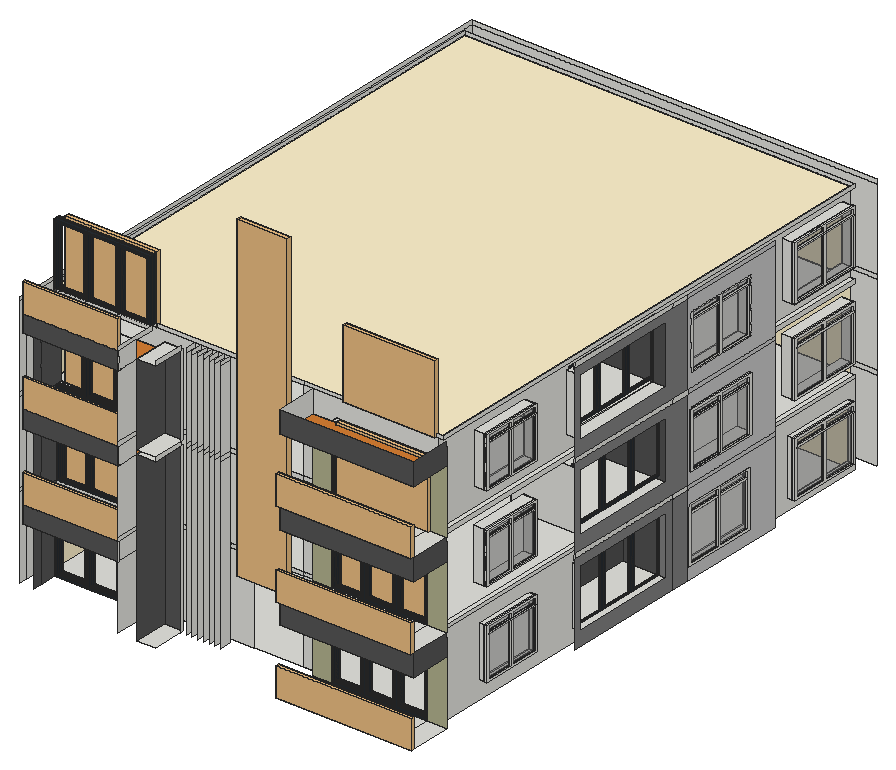
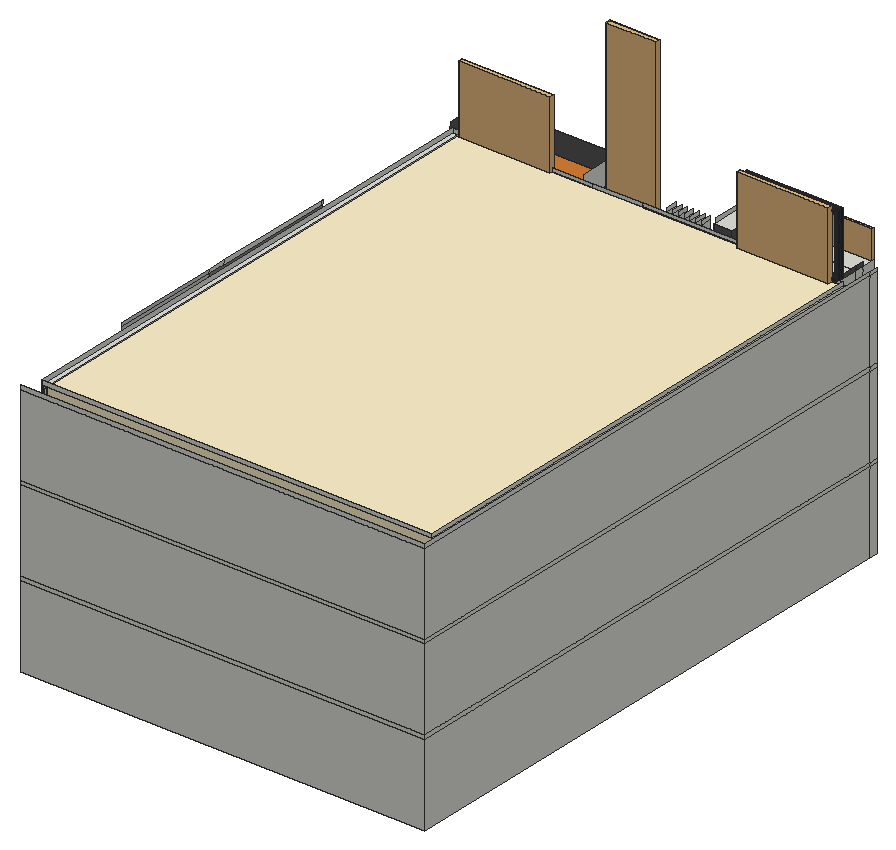
# SketchUp Ruby script. Lengths in inches.
U = 1.inch
M = Sketchup.active_model
def pt(a) = Geom::Point3d.new(a.map { |v| v * U })
def face(e, loops, mat)
  f = e.add_face(loops[0].map { |a| pt(a) })
  loops[1..].each { |l| e.add_face(l.map { |a| pt(a) }).erase! }
  f.material = f.back_material = mat if mat
  f
end
# faces: each face lists its corners as indices into pts; further lists are holes
def faces(e, pts, list, mat = nil) = list.each { |f| face(e, (f[0].is_a?(Array) ? f : [f]).map { |l| l.map { |i| pts[i] } }, mat) }
# xy, xz, yz: faces in a plane at the given z, y or x. An outline is a flat list of corners, or four numbers for a rectangle; further outlines are holes
def ring(l) = l.size == 4 ? [[l[0], l[1]], [l[2], l[1]], [l[2], l[3]], [l[0], l[3]]] : l.each_slice(2).to_a
def flat(e, list, mat, &to3) = list.each { |f| face(e, (f[0].is_a?(Array) ? f : [f]).map { |l| ring(l).map { |u, v| to3.(u, v) } }, mat) }
def xy(e, z, list, mat = nil) = flat(e, list, mat) { |x, y| [x, y, z] }
def xz(e, y, list, mat = nil) = flat(e, list, mat) { |x, z| [x, y, z] }
def yz(e, x, list, mat = nil) = flat(e, list, mat) { |y, z| [x, y, z] }
def lines(e, pts, list) = list.each { |a, b| e.add_line(pt(pts[a]), pt(pts[b])) }
# prism: a flat outline (further loops are holes) pulled along v
def prism(e, loops, v, mat = nil)
  f = face(e, loops, mat); d = Geom::Vector3d.new(v.map { |x| x * U })
  f.pushpull(f.normal.samedirection?(d) ? d.length : -d.length)
end
def box(e, o, s, mat = nil) = prism(e, [[o, [o[0] + s[0], o[1], o[2]], [o[0] + s[0], o[1] + s[1], o[2]], [o[0], o[1] + s[1], o[2]]]], [0, 0, s[2]], mat)
def at(x, y, z, deg = 0) = Geom::Transformation.translation(pt([x, y, z])) * Geom::Transformation.rotation(ORIGIN, Z_AXIS, deg.degrees)
def axes(o, x, y, z) = Geom::Transformation.new([*x, 0, *y, 0, *z, 0, *pt(o).to_a, 1])
def part(name) = M.definitions.add(name)
# library, detail: a bought-in or finely detailed component or shape, given as its bounding box
def library(name, o, s) = part(name).tap { |d| box(d.entities, o, s) }
def detail(e, o, s) = box(e.add_group.entities, o, s)
def put(e, d, t, mat = nil) = e.add_instance(d, t).tap { |i| i.material = mat if mat }
def group(e, t, mat = nil) = e.add_group.tap { |g| g.transformation = t; g.material = mat if mat }.entities
root = M.entities
M.materials.add("Wine2").color = [0, 0, 0]
M.materials["Wine2"].alpha = 0
M.materials.add("[0130_Gainsboro]").color = [39, 45, 50]
M.materials.add("[0133_Gray]").color = [128, 128, 128]
M.materials.add("[0135_DarkGray]1").color = [81, 81, 81]
M.materials.add("[Color D01]").color = [255, 242, 204]
M.materials.add("[Color E01]").color = [178, 178, 142]
M.materials.add("[Color M02]").color = [198, 198, 198]
M.materials.add("[Color M06]").color = [86, 86, 86]
M.materials.add("[Translucent Glass Gray]").color = [128, 128, 128]
M.materials["[Translucent Glass Gray]"].alpha = 0.5
M.materials.add("[Wood Bamboo]").color = [214, 127, 52]
c1 = library("Glass Railing",[0,0,0],[139.5,4.76,42])
c2 = part("Framed glazing panel")
xy(c2.entities,0,[[0,-0.98,43.07,0],[0,0,43.07,1.4]],"[0130_Gainsboro]")
xy(c2.entities,0.3,[[0.3,-1.43,42.77,-0.98]],"[0130_Gainsboro]")
xy(c2.entities,2.95,[[2.95,-1.43,40.12,-0.63],[2.95,-0.63,40.12,0],[2.95,0,40.12,0.64],[2.95,0.64,40.12,1.4]],"[0130_Gainsboro]")
xy(c2.entities,3.54,[[3.54,-0.63,39.53,0],[3.54,0,39.53,0.64]],"[0130_Gainsboro]")
xy(c2.entities,111.8125,[[3.54,-0.63,39.53,0],[3.54,0,39.53,0.64]],"[0130_Gainsboro]")
xy(c2.entities,112.4,[[2.95,-1.43,40.12,-0.63],[2.95,-0.63,40.12,0],[2.95,0,40.12,0.64],[2.95,0.64,40.12,1.4]],"[0130_Gainsboro]")
xy(c2.entities,115.05,[[0.3,-1.43,42.77,-0.98]],"[0130_Gainsboro]")
xy(c2.entities,115.35,[[0,-0.98,43.07,0],[0,0,43.07,1.4]],"[0130_Gainsboro]")
xz(c2.entities,-1.43,[[[0.3,0.3,42.77,115.05],[2.95,2.95,40.12,112.4]]],"[0130_Gainsboro]")
xz(c2.entities,-0.98,[[[0,0,43.07,115.35],[0.3,0.3,42.77,115.05]]],"[0130_Gainsboro]")
xz(c2.entities,-0.63,[[[2.95,2.95,40.12,112.4],[3.54,3.54,39.53,111.8125]]],"[0130_Gainsboro]")
xz(c2.entities,0,[[3.54,3.54,39.53,111.8125]],"Wine2")
xz(c2.entities,0,[[[0,0,43.07,115.35],[2.95,2.95,40.12,112.4]],[[2.95,2.95,40.12,112.4],[3.54,3.54,39.53,111.8125]]],"[0130_Gainsboro]")
xz(c2.entities,0.64,[[[2.95,2.95,40.12,112.4],[3.54,3.54,39.53,111.8125]]],"[0130_Gainsboro]")
xz(c2.entities,1.4,[[[0,0,43.07,115.35],[2.95,2.95,40.12,112.4]]],"[0130_Gainsboro]")
yz(c2.entities,0,[[-0.98,0,0,115.35],[0,0,1.4,115.35]],"[0130_Gainsboro]")
yz(c2.entities,0.3,[[-1.43,0.3,-0.98,115.05]],"[0130_Gainsboro]")
yz(c2.entities,2.95,[[-1.43,2.95,-0.63,112.4],[-0.63,2.95,0,112.4],[0,2.95,0.64,112.4],[0.64,2.95,1.4,112.4]],"[0130_Gainsboro]")
yz(c2.entities,3.54,[[-0.63,3.54,0,111.8125],[0,3.54,0.64,111.8125]],"[0130_Gainsboro]")
yz(c2.entities,39.53,[[-0.63,3.54,0,111.8125],[0,3.54,0.64,111.8125]],"[0130_Gainsboro]")
yz(c2.entities,40.12,[[-1.43,2.95,-0.63,112.4],[-0.63,2.95,0,112.4],[0,2.95,0.64,112.4],[0.64,2.95,1.4,112.4]],"[0130_Gainsboro]")
yz(c2.entities,42.77,[[-1.43,0.3,-0.98,115.05]],"[0130_Gainsboro]")
yz(c2.entities,43.07,[[-0.98,0,0,115.35],[0,0,1.4,115.35]],"[0130_Gainsboro]")
c3 = part("Glazing assembly")
put(c3.entities,c2,axes([90.57,1.43,0],[1.05148,0,0],[0,1,0],[0,0,1]))
put(c3.entities,c2,axes([0,1.43,0],[1.05148,0,0],[0,1,0],[0,0,1]))
put(c3.entities,c2,axes([45.29,1.43,0],[1.05148,0,0],[0,1,0],[0,0,1]))
c4 = part("Group\#3")
xy(c4.entities,0,[[0,0,32.48,1.97]])
xy(c4.entities,0.98,[[0.98,0,31.5,0.98],[0.98,0.98,31.5,1.97]])
xy(c4.entities,8.86,[[0.98,0,31.5,0.98],[0.98,0.98,31.5,1.97]])
xy(c4.entities,9.84,[[0,0,32.48,1.97]])
xz(c4.entities,0,[[[0,0,32.48,9.84],[0.98,0.98,31.5,8.86]]])
xz(c4.entities,0.98,[[0.98,0.98,31.5,8.86]],"[Translucent Glass Gray]")
xz(c4.entities,1.97,[[[0,0,32.48,9.84],[0.98,0.98,31.5,8.86]]])
yz(c4.entities,0,[[0,0,1.97,9.84]])
yz(c4.entities,0.98,[[0,0.98,0.98,8.86],[0.98,0.98,1.97,8.86]])
yz(c4.entities,31.5,[[0,0.98,0.98,8.86],[0.98,0.98,1.97,8.86]])
yz(c4.entities,32.48,[[0,0,1.97,9.84]])
c5 = part("Group\#4")
xy(c5.entities,0,[[0,0,32.48,1.97]])
xy(c5.entities,0.98,[[0.98,0,31.5,0.98],[0.98,0.98,31.5,1.97]])
xy(c5.entities,71.85,[[0.98,0,31.5,0.98],[0.98,0.98,31.5,1.97]])
xy(c5.entities,72.83,[[0,0,32.48,1.97]])
xz(c5.entities,0,[[[0,0,32.48,72.83],[0.98,0.98,31.5,71.85]]])
xz(c5.entities,0.98,[[0.98,0.98,31.5,71.85]],"[Translucent Glass Gray]")
xz(c5.entities,1.97,[[[0,0,32.48,72.83],[0.98,0.98,31.5,71.85]]])
yz(c5.entities,0,[[0,0,1.97,72.83]])
yz(c5.entities,0.98,[[0,0.98,0.98,71.85],[0.98,0.98,1.97,71.85]])
yz(c5.entities,31.5,[[0,0.98,0.98,71.85],[0.98,0.98,1.97,71.85]])
yz(c5.entities,32.48,[[0,0,1.97,72.83]])
c6 = part("FIXED+GLASS+WINDOW+WITH+TRANSOM")
g1 = group(c6.entities,at(0,0,0))
xy(g1,0,[[0,0,70.86,3.9375]])
xy(g1,1.97,[[1.97,0,34.45,0.98],[36.42,0,68.9,3.9375],[1.97,2.95,34.45,3.9375]])
xy(g1,86.61,[[1.97,0,34.45,3.9375],[34.45,0,36.42,3.9375],[36.42,0,68.9,3.9375]])
xy(g1,88.58,[[0,0,70.86,3.9375]])
xz(g1,0,[[[0,0,70.86,88.58],[1.97,1.97,34.45,86.61],[36.42,1.97,68.9,86.61]]])
xz(g1,3.9375,[[[0,0,70.86,88.58],[1.97,1.97,34.45,86.61],[36.42,1.97,68.9,86.61]]])
yz(g1,0,[[0,0,3.9375,88.58]])
yz(g1,1.97,[[0,1.97,3.9375,74.8],[0,76.77,3.9375,86.61]])
yz(g1,34.45,[[0,1.97,3.9375,86.61]])
yz(g1,36.42,[[0,1.97,3.9375,86.61]])
yz(g1,68.9,[[0,1.97,3.9375,86.61]])
yz(g1,70.86,[[0,0,3.9375,88.58]])
g2 = group(g1,at(1.97,0,74.8))
box(g2,[0,0,0],[66.93,3.9375,1.97])
put(g1,c4,at(1.97,0.98,76.77))
put(g1,c4,at(36.42,0.98,76.77))
put(g1,c5,at(1.97,0.98,1.97))
put(g1,c5,at(36.42,0.98,1.97))
c7 = library("Scandinavian Door w/ Glass Wall\#2",[-41.94,78.85,0],[6.47,62.99,82.68])
c8 = library("Group5_1",[-7.56,-66.38,0.11],[6.33,135.04,120.95])
xy(root,629.625,[[326.68,240.0625,354.04,290.5],[536.21,240.3125,563.32,301.625],[563.32,240.3125,704.2,310.82],[704.2,240.3125,733.4375,301.625],[157.82,301.625,298.7,310.82],
  [146.57,310.82,721.74,1067.8]])
xy(root,648.83,[[721.74,942.08,733.4375,1053.14]])
xy(root,649.38,[[721.74,750.25,733.4375,861.32]])
xy(root,651.41,[[670.36,546.17,721.74,704.54],[721.74,546.17,733.4375,704.54]])
xy(root,658.03,[[721.74,375.23,733.4375,467.6]])
xy(root,723.6875,[[563.32,301.625,704.2,310.82]])
xy(root,723.6875,[[157.82,240.3125,298.7,273.3125],[536.21,240.3125,733.4375,301.625],[157.82,273.3125,298.7,310.82]],"[Wood Bamboo]")
xy(root,730.08,[[721.74,942.08,733.4375,1053.14]])
xy(root,730.63,[[721.74,750.25,733.4375,861.32]])
xy(root,732.53,[[721.74,375.23,733.4375,467.6]])
xy(root,736.73,[[670.36,546.17,721.74,704.54],[721.74,546.17,733.4375,704.54]])
xy(root,749.625,[[157.82,240.3125,298.7,273.3125],[157.82,273.3125,298.7,301.625]])
xy(root,749.625,[[146.57,310.82,721.74,1067.8]],"[Color D01]")
xy(root,755.625,[[536.21,240.3125,563.32,301.625],[563.32,240.3125,704.2,310.82],[704.2,240.3125,733.4375,301.625],[157.82,301.625,298.7,310.82],[146.57,310.82,713.5,1067.8],
  [713.5,310.82,721.74,1067.8]])
xy(root,775.38,[[713.5,750.25,733.4375,861.32]])
xy(root,777.41,[[631.25,546.17,733.4375,704.54]])
xy(root,780.83,[[713.5,942.08,733.4375,1053.14]])
xy(root,784.03,[[713.5,375.23,733.4375,467.6]])
xy(root,849.6875,[[563.32,301.625,704.2,310.82]])
xy(root,849.6875,[[157.82,240.3125,298.7,273.3125],[536.21,240.3125,733.4375,301.625],[157.82,273.3125,298.7,310.82]],"[Wood Bamboo]")
xy(root,856.63,[[713.5,750.25,733.4375,861.32]])
xy(root,858.53,[[713.5,375.23,733.4375,467.6]])
xy(root,862.08,[[713.5,942.08,733.4375,1053.14]])
xy(root,862.73,[[631.25,546.17,733.4375,704.54]])
xy(root,875.625,[[326.68,240.0625,354.04,290.5],[157.82,240.3125,298.7,273.3125],[157.82,273.3125,298.7,301.625],[713.5,310.82,721.74,1067.8]])
xy(root,875.625,[[146.57,310.82,713.5,1067.8]],"[Color D01]")
xy(root,881.625,[[326.68,240.0625,354.04,290.5],[536.21,240.3125,563.32,301.625],[563.32,240.3125,704.2,310.82],[704.2,240.3125,733.4375,301.625],[157.82,301.625,298.7,310.82],
  [146.57,310.82,713.5,1067.8],[713.5,310.82,721.74,1067.8]])
xy(root,901.38,[[713.5,750.25,733.4375,861.32]])
xy(root,903.41,[[631.25,546.17,713.5,704.54],[713.5,546.17,733.4375,704.54]])
xy(root,906.83,[[713.5,942.08,733.4375,1053.14]])
xy(root,910.03,[[713.5,375.23,733.4375,467.6]])
xy(root,975.6875,[[563.32,301.625,704.2,310.82]])
xy(root,975.6875,[[157.82,240.3125,298.7,273.3125],[536.21,240.3125,733.4375,301.625],[157.82,273.3125,298.7,310.82]],"[Wood Bamboo]")
xy(root,982.63,[[713.5,750.25,733.4375,861.32]])
xy(root,984.53,[[713.5,375.23,733.4375,467.6]])
xy(root,988.08,[[713.5,942.08,733.4375,1053.14]])
xy(root,988.73,[[631.25,546.17,713.5,704.54],[713.5,546.17,733.4375,704.54]])
xy(root,1001.625,[[326.68,240.0625,354.04,290.5],[157.82,240.3125,298.7,273.3125],[157.82,273.3125,298.7,301.625],[713.5,310.82,721.74,1067.8]])
xy(root,1001.625,[[146.57,310.82,713.5,1067.8]],"[Color D01]")
xz(root,240.3125,[[157.82,723.6875,298.7,749.625],[536.21,723.6875,733.4375,755.625],[157.82,849.6875,298.7,875.625],[536.21,849.6875,733.4375,881.625],[157.82,975.6875,298.7,1001.625],
  [536.21,975.6875,733.4375,1007.625]],"[Color M06]")
xz(root,273.3125,[[157.82,723.6875,298.7,749.625],[157.82,849.6875,298.7,875.625],[157.82,975.6875,298.7,1001.625]])
xz(root,290.5,[[326.68,629.625,354.04,875.625],[326.68,881.625,354.04,1001.625]],"[Color M06]")
xz(root,301.625,[[157.82,749.625,298.7,755.625],[157.82,875.625,298.7,881.625],[157.82,1001.625,298.7,1007.625]])
xz(root,301.625,[[536.21,629.625,563.32,723.6875],[704.2,629.625,733.4375,723.6875],[536.21,755.625,563.32,849.6875],[704.2,755.625,733.4375,849.6875],[536.21,881.625,563.32,975.6875],
  [704.2,881.625,733.4375,975.6875]],"[Color E01]")
xz(root,310.82,[[146.57,629.625,146.57,749.625,442.42,749.625,442.42,629.625,298.7,629.625,298.7,723.6875,157.82,723.6875,157.82,629.625],[514.85,629.625,514.85,749.625,721.74,749.625,721.74,629.625,704.2,629.625,704.2,723.6875,563.32,723.6875,563.32,629.625],[146.57,749.625,442.42,755.625],[442.42,749.625,514.85,755.625],[514.85,749.625,721.74,755.625],
  [146.57,755.625,146.57,875.625,442.42,875.625,442.42,755.625,298.7,755.625,298.7,849.6875,157.82,849.6875,157.82,755.625],[514.85,755.625,514.85,875.625,713.5,875.625,713.5,755.625,704.2,755.625,704.2,849.6875,563.32,849.6875,563.32,755.625],[146.57,875.625,442.42,881.625],[442.42,875.625,514.85,881.625],[514.85,875.625,721.74,881.625],
  [146.57,881.625,146.57,1001.625,442.42,1001.625,442.42,881.625,298.7,881.625,298.7,975.6875,157.82,975.6875,157.82,881.625],[514.85,881.625,514.85,1001.625,713.5,1001.625,713.5,881.625,704.2,881.625,704.2,975.6875,563.32,975.6875,563.32,881.625],[146.57,1001.625,442.42,1007.625],[442.42,1001.625,514.85,1007.625],[514.85,1001.625,721.74,1007.625]])
xz(root,375.23,[[721.74,658.03,733.4375,732.53],[713.5,784.03,733.4375,858.53],[713.5,910.03,733.4375,984.53]])
xz(root,467.6,[[721.74,658.03,733.4375,732.53],[713.5,784.03,733.4375,858.53],[713.5,910.03,733.4375,984.53]])
xz(root,546.17,[[670.36,651.41,721.74,736.73],[721.74,651.41,733.4375,736.73],[631.25,777.41,733.4375,862.73],[631.25,903.41,713.5,988.73],[713.5,903.41,733.4375,988.73]])
xz(root,704.54,[[721.74,651.41,733.4375,736.73]],"[0133_Gray]")
xz(root,704.54,[[670.36,651.41,721.74,736.73],[631.25,777.41,733.4375,862.73],[631.25,903.41,713.5,988.73],[713.5,903.41,733.4375,988.73]],"[0135_DarkGray]1")
xz(root,750.25,[[721.74,649.38,733.4375,730.63],[713.5,775.38,733.4375,856.63],[713.5,901.38,733.4375,982.63]])
xz(root,861.32,[[721.74,649.38,733.4375,730.63],[713.5,775.38,733.4375,856.63],[713.5,901.38,733.4375,982.63]])
xz(root,942.08,[[721.74,648.83,733.4375,730.08],[713.5,780.83,733.4375,862.08],[713.5,906.83,733.4375,988.08]])
xz(root,1053.14,[[721.74,648.83,733.4375,730.08],[713.5,780.83,733.4375,862.08],[713.5,906.83,733.4375,988.08]])
xz(root,1067.8,[[146.57,749.625,721.74,755.625],[146.57,875.625,721.74,881.625],[146.57,1001.625,721.74,1007.625]])
xz(root,1067.8,[[146.57,629.625,721.74,749.625],[146.57,755.625,713.5,875.625],[146.57,881.625,713.5,1001.625]],"[Color D01]")
xz(root,1091.875,[[137.375,629.625,733.4375,749.625],[137.375,749.625,733.4375,755.625],[137.375,755.625,733.4375,875.625],[137.375,875.625,733.4375,881.625],[137.375,881.625,733.4375,1001.625],
  [137.375,1001.625,733.4375,1007.625]])
yz(root,137.375,[[261.5,629.625,273.3125,749.625],[273.3125,629.625,1091.875,749.625],[261.5,749.625,273.3125,755.625],[273.3125,749.625,1091.875,755.625],[261.5,755.625,273.3125,875.625],
  [273.3125,755.625,1091.875,875.625],[261.5,875.625,273.3125,881.625],[273.3125,875.625,1091.875,881.625],[261.5,881.625,273.3125,1001.625],[273.3125,881.625,1091.875,1001.625],
  [261.5,1001.625,273.3125,1007.625],[273.3125,1001.625,1091.875,1007.625]])
yz(root,146.57,[[310.82,749.625,1067.8,755.625],[310.82,875.625,1067.8,881.625],[310.82,1001.625,1067.8,1007.625]])
yz(root,146.57,[[310.82,629.625,1067.8,749.625],[310.82,755.625,1067.8,875.625],[310.82,881.625,1067.8,1001.625]],"[Color D01]")
yz(root,157.82,[[240.3125,723.6875,261.5,749.625],[261.5,723.6875,273.3125,749.625],[240.3125,849.6875,261.5,875.625],[261.5,849.6875,273.3125,875.625],[240.3125,975.6875,261.5,1001.625],
  [261.5,975.6875,273.3125,1001.625]])
yz(root,157.82,[[261.5,629.625,273.3125,723.6875],[273.3125,629.625,310.82,723.6875],[261.5,749.625,273.3125,755.625],[273.3125,749.625,301.625,755.625],[261.5,755.625,273.3125,849.6875],
  [273.3125,755.625,310.82,849.6875],[261.5,875.625,273.3125,881.625],[273.3125,875.625,301.625,881.625],[261.5,881.625,273.3125,975.6875],[273.3125,881.625,310.82,975.6875],
  [261.5,1001.625,273.3125,1007.625],[273.3125,1001.625,301.625,1007.625]],"[Color M06]")
yz(root,298.7,[[240.0625,629.625,310.82,723.6875],[240.0625,723.6875,240.3125,749.625],[240.3125,723.6875,273.3125,749.625],[240.0625,749.625,301.625,755.625],[240.0625,755.625,310.82,849.6875],
  [240.0625,849.6875,240.3125,875.625],[240.3125,849.6875,273.3125,875.625],[240.0625,875.625,301.625,881.625],[240.0625,881.625,310.82,975.6875],[240.0625,975.6875,240.3125,1001.625],
  [240.3125,975.6875,273.3125,1001.625],[240.0625,1001.625,301.625,1007.625]])
yz(root,326.68,[[240.0625,629.625,290.5,875.625],[240.0625,881.625,290.5,1001.625]],"[Color M06]")
yz(root,354.04,[[285.875,629.625,290.5,875.625],[240.0625,875.625,285.875,881.625],[285.875,881.625,290.5,1001.625],[240.0625,1001.625,285.875,1007.625]])
yz(root,362.47,[[285.875,629.625,301.625,875.625],[285.875,875.625,301.625,881.625],[285.875,881.625,301.625,1001.625],[285.875,1001.625,301.625,1007.625]])
yz(root,370.91,[[285.875,629.625,301.625,875.625],[285.875,875.625,301.625,881.625],[285.875,881.625,301.625,1001.625],[285.875,1001.625,301.625,1007.625]])
yz(root,379.35,[[285.875,629.625,301.625,875.625],[285.875,875.625,301.625,881.625],[285.875,881.625,301.625,1001.625],[285.875,1001.625,301.625,1007.625]])
yz(root,387.79,[[285.875,629.625,301.625,875.625],[285.875,875.625,301.625,881.625],[285.875,881.625,301.625,1001.625],[285.875,1001.625,301.625,1007.625]])
yz(root,396.22,[[285.875,629.625,301.625,875.625],[285.875,875.625,301.625,881.625],[285.875,881.625,301.625,1001.625],[285.875,1001.625,301.625,1007.625]])
yz(root,404.66,[[285.875,629.625,301.625,875.625],[285.875,875.625,301.625,881.625],[285.875,881.625,301.625,1001.625],[285.875,1001.625,301.625,1007.625]])
yz(root,413.1,[[285.875,629.625,301.625,875.625],[285.875,875.625,301.625,881.625],[285.875,881.625,301.625,1001.625],[285.875,1001.625,301.625,1007.625]])
yz(root,536.21,[[240.3125,723.6875,301.625,755.625],[240.3125,849.6875,301.625,881.625],[240.3125,975.6875,301.625,1007.625]])
yz(root,563.32,[[301.625,629.625,310.82,723.6875],[301.625,755.625,310.82,849.6875],[301.625,881.625,310.82,975.6875]])
yz(root,631.25,[[546.17,777.41,704.54,862.73],[546.17,903.41,704.54,988.73]],"[0135_DarkGray]1")
yz(root,670.36,[[546.17,651.41,704.54,736.73]],"[0135_DarkGray]1")
yz(root,704.2,[[301.625,629.625,310.82,723.6875],[301.625,755.625,310.82,849.6875],[301.625,881.625,310.82,975.6875]])
yz(root,713.5,[[[310.82,881.625,1067.8,1001.625],[546.17,903.41,704.54,988.73],[750.25,901.38,861.32,982.63],[942.08,906.83,1053.14,988.08],[375.23,910.03,467.6,984.53]]])
yz(root,721.74,[[[310.82,629.625,1067.8,749.625],[546.17,651.41,704.54,736.73],[750.25,649.38,861.32,730.63],[942.08,648.83,1053.14,730.08],[375.23,658.03,467.6,732.53]],[310.82,749.625,1067.8,755.625],[310.82,875.625,1067.8,881.625],[310.82,1001.625,1067.8,1007.625]])
yz(root,733.4375,[[534.42,749.625,537.75,755.625],[537.75,749.625,716.73,755.625],[716.73,749.625,744.22,755.625],[534.42,875.625,537.75,881.625],[537.75,875.625,716.73,881.625],
  [716.73,875.625,744.22,881.625],[534.42,1001.625,537.75,1007.625],[537.75,1001.625,716.73,1007.625],[716.73,1001.625,744.22,1007.625]])
yz(root,733.4375,[[[537.75,629.625,716.73,749.625],[546.17,651.41,704.54,736.73]],[716.73,629.625,744.22,749.625],[[537.75,755.625,744.22,875.625],[546.17,777.41,704.54,862.73]],[[537.75,881.625,744.22,1001.625],[546.17,903.41,704.54,988.73]]],"[0133_Gray]")
yz(root,733.4375,[[[744.22,629.625,904.3,749.625],[750.25,649.38,861.32,730.63]],[744.22,749.625,904.3,755.625],[[744.22,755.625,904.3,875.625],[750.25,775.38,861.32,856.63]],[744.22,875.625,904.3,881.625],[[744.22,881.625,904.3,1001.625],[750.25,901.38,861.32,982.63]],
  [744.22,1001.625,904.3,1007.625]],"[Color M02]")
yz(root,733.4375,[[240.3125,723.6875,301.625,723.6875,301.625,749.625,300.15,749.625,300.15,755.625,240.3125,755.625],[240.3125,849.6875,301.625,849.6875,301.625,875.625,300.15,875.625,300.15,881.625,240.3125,881.625],[240.3125,975.6875,301.625,975.6875,301.625,1001.625,300.15,1001.625,300.15,1007.625,240.3125,1007.625]],"[Color M06]")
p = [[733.4375,301.625,875.625],[730,301.625,875.625],[733.4375,300.15,881.625],[733.4375,301.625,749.625],[678.8125,301.625,749.625],[733.4375,300.15,755.625]]
lines(root,p,[[0,1],[1,2],[3,4],[4,5]])
put(root,c1,axes([534.23,236.51,628.93],[1.428,0,0],[0,1,0],[0,0,1]),"[Color E01]")
put(root,c3,axes([157.82,310.82,629.625],[1.03691,0,0],[0,-4,0],[0,0,0.80657]))
put(root,c3,axes([563.32,312.95,629.625],[1.03691,0,0],[0,-4,0],[0,0,0.80657]))
put(root,c6,axes([733.4375,747.17,647.58],[0,1.56726,0],[-1,0,0],[0,0,0.91722]))
put(root,c6,axes([733.4375,942.08,648.83],[0,1.56726,0],[-1,0,0],[0,0,0.91722]))
put(root,c3,axes([722.64,549.85,648.86],[0,1.17066,0],[-1.13,0,0],[0,0,0.72061]))
put(root,c6,axes([733.4375,375.23,658.03],[0,1.30355,0],[-1,0,0],[0,0,0.84102]))
put(root,c7,axes([350.96,243.91,738.3],[0,-1,0],[1.16,0,0],[0,0,5.69]))
put(root,c1,at(157.82,240.3125,749.625))
put(root,c8,axes([635.54,309.6,749.71],[0,-1,0],[1,0,0],[0,0,0.83156]))
put(root,c8,axes([234.03,306.51,750.87],[0,-1,0],[1,0,0],[0,0,0.83156]))
put(root,c3,axes([157.82,312.95,755.625],[1.03691,0,0],[0,-4,0],[0,0,0.80657]))
put(root,c3,axes([563.32,312.95,755.625],[1.03691,0,0],[0,-4,0],[0,0,0.80657]))
put(root,c1,axes([534.23,235.55,755.625],[1.428,0,0],[0,1,0],[0,0,1]))
put(root,c6,axes([736.39,747.17,773.58],[0,1.56726,0],[-1,0,0],[0,0,0.91722]))
put(root,c6,axes([733.4375,942.08,780.83],[0,1.56726,0],[-1,0,0],[0,0,0.91722]))
put(root,c3,axes([722.64,549.85,781.36],[0,1.17066,0],[-1.13,0,0],[0,0,0.72061]))
put(root,c6,axes([733.4375,375.23,784.03],[0,1.30355,0],[-1,0,0],[0,0,0.84102]))
put(root,c8,axes([230.04,309.6,875.02],[0,-1,0],[1,0,0],[0,0,0.83156]))
put(root,c1,at(157.82,240.3125,875.625))
put(root,c8,axes([639.47,297.16,878.26],[0,-1,0],[1,0,0],[0,0,0.83156]))
put(root,c3,axes([153.96,309.91,878.77],[1.03691,0,0],[0,-4,0],[0,0,0.80657]),"[Color M06]")
put(root,c3,axes([563.32,312.95,881.625],[1.03691,0,0],[0,-4,0],[0,0,0.80657]))
put(root,c1,axes([534.23,235.55,882.6875],[1.428,0,0],[0,1,0],[0,0,1]))
put(root,c6,axes([733.4375,750.25,901.38],[0,1.56726,0],[-1,0,0],[0,0,0.91722]))
put(root,c3,axes([714.4,549.85,907.8],[0,1.17066,0],[-1.13,0,0],[0,0,0.72061]))
put(root,c6,axes([733.4375,942.08,908.15],[0,1.56726,0],[-1,0,0],[0,0,0.91722]))
put(root,c6,axes([733.4375,375.23,910.03],[0,1.30355,0],[-1,0,0],[0,0,0.84102]))
put(root,c8,axes([230.04,309.6,1001.02],[0,-1,0],[1,0,0],[0,0,0.83156]))
put(root,c1,at(157.82,240.3125,1001.625))
put(root,c8,axes([641.4375,307.34,1002.06],[0,-1,0],[1,0,0],[0,0,0.83156]))
put(root,c3,axes([154.6,312.95,1005.24],[1.03691,0,0],[0,-4,0],[0,0,0.80657]))
